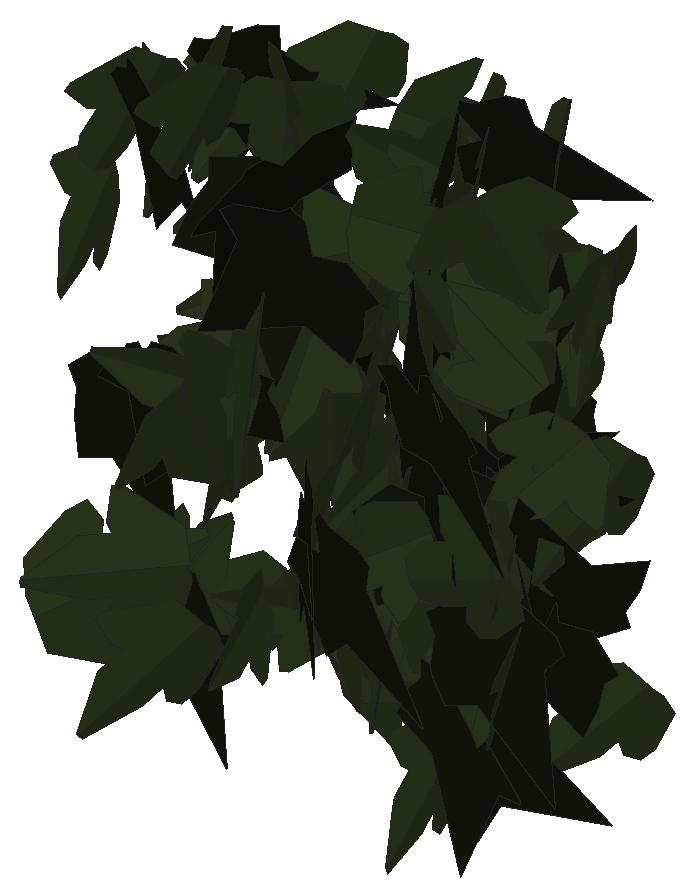
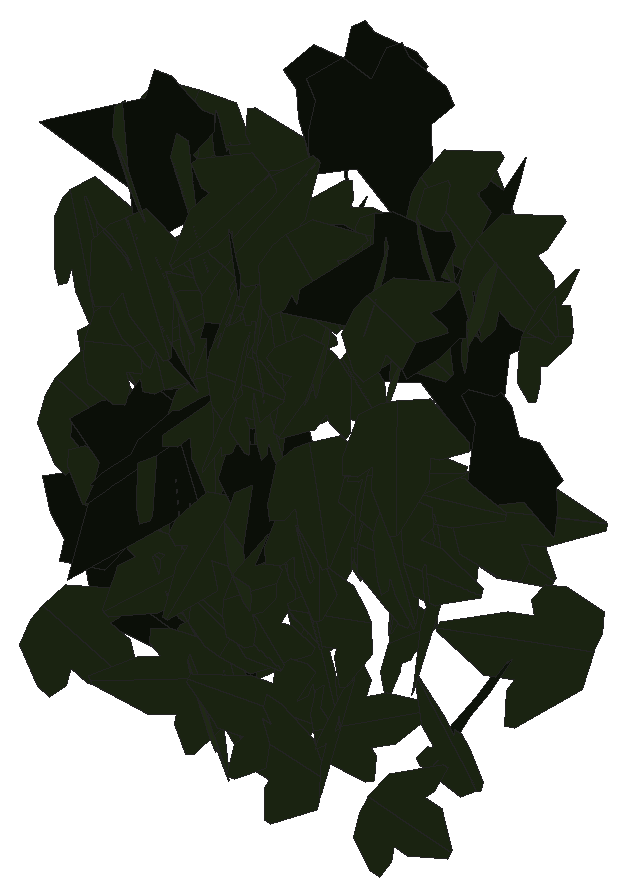
# SketchUp Ruby script. Lengths in inches.
U = 1.inch
M = Sketchup.active_model
def pt(a) = Geom::Point3d.new(a.map { |v| v * U })
def face(e, loops, mat)
  f = e.add_face(loops[0].map { |a| pt(a) })
  loops[1..].each { |l| e.add_face(l.map { |a| pt(a) }).erase! }
  f.material = f.back_material = mat if mat
  f
end
# faces: each face lists its corners as indices into pts; further lists are holes
def faces(e, pts, list, mat = nil) = list.each { |f| face(e, (f[0].is_a?(Array) ? f : [f]).map { |l| l.map { |i| pts[i] } }, mat) }
# xy, xz, yz: faces in a plane at the given z, y or x. An outline is a flat list of corners, or four numbers for a rectangle; further outlines are holes
def ring(l) = l.size == 4 ? [[l[0], l[1]], [l[2], l[1]], [l[2], l[3]], [l[0], l[3]]] : l.each_slice(2).to_a
def flat(e, list, mat, &to3) = list.each { |f| face(e, (f[0].is_a?(Array) ? f : [f]).map { |l| ring(l).map { |u, v| to3.(u, v) } }, mat) }
def xy(e, z, list, mat = nil) = flat(e, list, mat) { |x, y| [x, y, z] }
def xz(e, y, list, mat = nil) = flat(e, list, mat) { |x, z| [x, y, z] }
def yz(e, x, list, mat = nil) = flat(e, list, mat) { |y, z| [x, y, z] }
def lines(e, pts, list) = list.each { |a, b| e.add_line(pt(pts[a]), pt(pts[b])) }
# prism: a flat outline (further loops are holes) pulled along v
def prism(e, loops, v, mat = nil)
  f = face(e, loops, mat); d = Geom::Vector3d.new(v.map { |x| x * U })
  f.pushpull(f.normal.samedirection?(d) ? d.length : -d.length)
end
def box(e, o, s, mat = nil) = prism(e, [[o, [o[0] + s[0], o[1], o[2]], [o[0] + s[0], o[1] + s[1], o[2]], [o[0], o[1] + s[1], o[2]]]], [0, 0, s[2]], mat)
def at(x, y, z, deg = 0) = Geom::Transformation.translation(pt([x, y, z])) * Geom::Transformation.rotation(ORIGIN, Z_AXIS, deg.degrees)
def axes(o, x, y, z) = Geom::Transformation.new([*x, 0, *y, 0, *z, 0, *pt(o).to_a, 1])
def part(name) = M.definitions.add(name)
# library, detail: a bought-in or finely detailed component or shape, given as its bounding box
def library(name, o, s) = part(name).tap { |d| box(d.entities, o, s) }
def detail(e, o, s) = box(e.add_group.entities, o, s)
def put(e, d, t, mat = nil) = e.add_instance(d, t).tap { |i| i.material = mat if mat }
def group(e, t, mat = nil) = e.add_group.tap { |g| g.transformation = t; g.material = mat if mat }.entities
root = M.entities
M.materials.add("efeu1").color = [18, 25, 13]
M.materials.add("efeu2").color = [43, 57, 29]
c1 = part("ivyleaf_10")
p = [[0,0.5,-0.03],[-0.0625,2.02,-0.43],[-0.19,2.01,-0.46],[-0.54,1.05,-0.29],[-0.52,0.625,-0.18],[-0.83,0.76,-0.28],
  [-1.16,0.64,-0.33],[-1.15,0.33,-0.24],[-0.77,-0.39,0.02],[-0.3,-0.51,0.16],[0.04,-0.48,0.23],[-0.02,2.01,-0.4375],
  [-0.06,2.01,-0.43],[0.04,-0.49,0.23],[0.67,-0.49,0.14],[1.38,0.36,-0.2],[1.375,0.51,-0.24],[0.81,0.65,-0.19],
  [0.62,0.59,-0.15],[0.6,1.09,-0.28],[0.5,1.23,-0.31]]
faces(c1.entities,p,[[0,1,2,3,4,5,6,7,8,9,10],[11,12,0,13,14,15,16,17,18,19,20]],"efeu2")
c2 = part("ivyleaf_9")
p = [[1.54,2.16,1.25],[1.36,2.04,1.19],[-0.21,0.99,0.68],[-0.71,1.11,0.82],[-0.85,0.86,0.67],[-0.8,0.17,0.21],
  [-0.9,-0.01,0.1],[-0.67,-0.16,-0.02],[-0.08,-0.08,-0.05],[-0.03,-0.6,-0.4],[0.65,-0.88,-0.66],[0.83,-0.6,-0.49],
  [1.29,-0.42,-0.43],[1.8125,-0.07,-0.26],[1.21,0.44,0.15]]
faces(c2.entities,p,[[0,1,2,3,4,5,6,7,8,9,10,11,12,13,14]],"efeu1")
put(root,c1,axes([513.32,135.32,171.68],[-0.08732,-0.65374,0.43706],[-0.02249,-0.43749,-0.65888],[0.78606,-0.08514,0.0297]))
put(root,c1,axes([513.06,134.78,170.35],[-0.06101,-0.33846,0.66501],[0.36152,-0.5971,-0.27073],[0.65277,0.29906,0.21209]))
put(root,c1,axes([513.72,136.18,166.54],[-0.09693,0.07568,0.7615],[-0.51086,0.5651,-0.12118],[-0.56976,-0.51956,-0.02089]))
put(root,c1,axes([513.16,136.26,164.39],[0.50718,-0.21012,-0.38853],[0.35496,-0.15822,0.54892],[-0.2629,-0.619,-0.00842]))
put(root,c1,axes([513.18,136.01,170.99],[-0.24057,-0.00862,0.63768],[0.5315,-0.37936,0.19539],[0.35244,0.56621,0.14061]))
put(root,c1,axes([513.66,137.22,164],[-0.17056,-0.41151,0.50788],[-0.01949,-0.52144,-0.42905],[0.65338,-0.12298,0.11978]))
put(root,c1,axes([514.2,136.55,167.49],[0.09159,0.0185,-0.7632],[-0.75052,0.14293,-0.0866],[0.13978,0.75527,0.03508]))
put(root,c1,axes([513.24,133.97,165.2],[0.19421,0.17082,-0.85137],[0.64383,0.55707,0.25864],[0.58266,-0.67248,-0.00201]))
put(root,c1,axes([513.79,136.84,169.625],[-0.37954,-0.60035,-0.04],[0.01676,0.03673,-0.71024],[0.60145,-0.37987,-0.00545]))
put(root,c1,axes([514.01,136.83,171.28],[-0.35701,-0.40739,0.47497],[-0.10446,-0.50037,-0.50768],[0.61697,-0.32045,0.18889]))
put(root,c1,axes([513.93,136.76,167.95],[0.13667,-0.66248,0.06443],[0.01464,-0.06276,-0.67643],[0.66544,0.13745,0.00165]))
put(root,c1,axes([514.35,136.03,168.1],[-0.11845,-0.06289,0.67388],[-0.43804,-0.51439,-0.125],[0.51593,-0.45116,0.04858]))
put(root,c2,axes([513.64,135.52,164.69],[0.32318,-0.69175,0.08443],[0.0373,-0.07576,-0.76352],[0.69588,0.32532,0.00172]))
put(root,c1,axes([514.35,136.75,168.73],[0.0879,0.09809,-0.65288],[-0.4716,-0.4516,-0.13134],[-0.46203,0.47962,0.00986]))
put(root,c1,axes([514.0625,135.82,172.1],[0.3082,-0.50599,0.35522],[0.20219,-0.29258,-0.5922],[0.58423,0.36819,0.01756]))
put(root,c2,axes([513.78,136.0625,171.59],[0.13494,0.26931,-0.70933],[0.27273,0.65509,0.3006],[0.70802,-0.30367,0.0194]))
put(root,c2,axes([513.86,134.19,168.27],[-0.28502,-0.09388,-0.70569],[0.66464,0.23729,-0.30001],[0.2551,-0.72314,-0.00683]))
put(root,c2,axes([513.89,134.9,171.41],[0.08524,-0.47252,0.60804],[0.14853,-0.59018,-0.47946],[0.75559,0.16932,0.02566]))
put(root,c1,axes([514.42,136.36,169.05],[-0.25689,0.64643,0.18666],[-0.08928,0.16529,-0.69528],[-0.66689,-0.27114,0.02118]))
put(root,c1,axes([514.54,135.01,172.07],[-0.00408,-0.68886,0.41079],[0.01597,-0.41078,-0.68869],[0.80189,0.00468,0.0158]))
put(root,c1,axes([514.97,133.48,166.45],[-0.04546,-0.04195,0.78348],[-0.47666,-0.6219,-0.06095],[0.62322,-0.4787,0.01053]))
put(root,c1,axes([514.625,135.36,167.27],[0.1349,-0.53892,-0.51614],[-0.0178,0.52204,-0.54972],[0.746,0.10991,0.08022]))
put(root,c1,axes([514.82,136.28,171.54],[-0.52337,-0.46039,0.09507],[-0.06521,-0.06981,-0.69698],[0.46556,-0.52733,0.00926]))
put(root,c1,axes([515.08,136.48,164.51],[-0.13673,0.03474,-0.62065],[-0.56309,-0.27614,0.1086],[-0.26334,0.57241,0.09006]))
put(root,c1,axes([514.47,135.98,170.16],[-0.25384,0.46249,-0.49972],[0.2253,-0.44622,-0.52742],[-0.64254,-0.33918,0.01248]))
put(root,c1,axes([514.51,136.41,171.78],[-0.41464,0.50002,-0.3271],[0.21653,-0.24533,-0.64952],[-0.55689,-0.46769,-0.009]))
put(root,c1,axes([514.95,136.55,164.92],[-0.29166,0.60031,0.10335],[-0.0587,0.08635,-0.66724],[-0.6063,-0.29713,0.01489]))
put(root,c1,axes([514.53,136.92,166.48],[-0.20723,0.09072,-0.63142],[0.56466,-0.2828,-0.22595],[-0.29679,-0.60139,0.011]))
put(root,c1,axes([515.11,136.86,167.78],[-0.40097,-0.54568,-0.01251],[0.00994,0.00822,-0.67715],[0.54573,-0.40108,0.00314]))
put(root,c1,axes([515.16,136.9,168.5625],[-0.30215,-0.6049,0.05545],[-0.02207,-0.05096,-0.67616],[0.60704,-0.30294,0.00301]))
put(root,c1,axes([515.2,137.2,171.93],[-0.29718,-0.49884,0.3104],[-0.05496,-0.32272,-0.57126],[0.58495,-0.28376,0.10402]))
put(root,c1,axes([515.21,135.11,165.18],[-0.03071,0.2233,-0.60377],[-0.00677,-0.60453,-0.22324],[-0.6437,-0.0043,0.03115]))
put(root,c1,axes([515.7,136.23,165.4375],[-0.32304,0.10404,0.5461],[-0.51564,0.17997,-0.33931],[-0.20776,-0.60844,-0.00699]))
put(root,c2,axes([515.59,133.45,169.28],[0.32299,0.46235,-0.55271],[-0.34821,-0.43013,-0.5633],[-0.63087,0.47412,0.02794]))
put(root,c1,axes([515.45,136.24,167.52],[-0.11325,-0.62591,-0.07851],[0.0108,0.07783,-0.63607],[0.63073,-0.11372,-0.0032]))
put(root,c1,axes([515.71,132.97,165.87],[-0.18062,-0.49797,0.59155],[-0.21017,-0.55299,-0.52968],[0.74413,-0.27705,-0.00602]))
put(root,c1,axes([515.31,136.57,169.84],[-0.57023,0.08825,-0.28166],[0.27161,-0.08298,-0.57587],[-0.11555,-0.63057,0.03637]))
put(root,c1,axes([515.65,136.75,167.36],[0.46985,-0.55043,-0.28111],[-0.18585,0.21094,-0.72368],[0.58945,0.50525,-0.00411]))
put(root,c1,axes([515.5625,136.34,170.16],[-0.47216,0.42684,-0.06049],[0.04122,-0.0446,-0.63647],[-0.42913,-0.47392,0.00542]))
put(root,c1,axes([516.16,133.28,169.33],[-0.20729,0.04473,-0.76954],[-0.74755,-0.20609,0.18938],[-0.18807,0.76986,0.09541]))
put(root,c2,axes([515.62,135.06,171.03],[-0.44138,-0.52209,-0.37281],[0.2329,0.29124,-0.6836],[0.59776,-0.49898,-0.00893]))
put(root,c1,axes([515.98,135.15,169.04],[0.21101,0.533,-0.30857],[-0.14739,-0.273,-0.57234],[-0.59798,0.25537,0.03218]))
put(root,c1,axes([515.54,136.78,163.85],[0.07508,-0.00656,-0.7683],[0.72273,-0.26137,0.07286],[-0.26074,-0.72636,-0.01928]))
put(root,c1,axes([515.95,136.4,166.77],[0.5732,-0.198,0.21383],[0.20355,-0.06563,-0.60641],[0.20855,0.60825,0.00417]))
put(root,c1,axes([516.05,137.36,166.48],[-0.03952,-0.15495,0.62079],[0.22707,-0.58488,-0.13153],[0.59818,0.21178,0.09095]))
put(root,c1,axes([516.17,135.27,167.16],[0.32619,-0.64833,0.21678],[0.1042,-0.19024,-0.72573],[0.67563,0.34236,0.00727]))
put(root,c1,axes([516.24,136.51,169.08],[0.16798,-0.62768,0.07538],[0.0277,-0.07061,-0.64971],[0.63158,0.17004,0.00844]))
put(root,c1,axes([516.5,135.98,169.89],[-0.58682,-0.11813,0.23916],[-0.2272,-0.08145,-0.59771],[0.13976,-0.62843,0.03251]))
put(root,c2,axes([515.68,136.8,167.73],[0.3406,-0.33455,0.60485],[0.41726,-0.43806,-0.47726],[0.55105,0.53848,-0.01247]))
put(root,c1,axes([515.9,136.45,164.3],[0.28401,0.23927,-0.69912],[0.54287,0.44057,0.37132],[0.50131,-0.61264,-0.00601]))
put(root,c1,axes([516.31,136.36,167.06],[0.04832,0.1535,-0.66955],[-0.12338,-0.65835,-0.15984],[-0.67575,0.13118,-0.01869]))
put(root,c1,axes([516.62,136.77,165.52],[-0.60869,-0.21908,-0.35197],[-0.31753,-0.15565,0.64601],[-0.26655,0.68568,0.03419]))
put(root,c1,axes([516.89,136.59,169.25],[-0.10985,0.12575,-0.71735],[-0.59963,0.39611,0.16126],[0.41333,0.60807,0.0433]))
put(root,c1,axes([516.3,137.07,167.19],[0.26297,-0.52173,0.42454],[0.19984,-0.37465,-0.5842],[0.64227,0.33019,0.00795]))
put(root,c1,axes([516.0625,136.95,170.03],[0.1598,-0.21747,0.57718],[0.49507,-0.31039,-0.25402],[0.36787,0.51218,0.09113]))
put(root,c1,axes([516.73,134.9,170.74],[-0.10812,0.0104,0.6499],[-0.25929,-0.60483,-0.03346],[0.59603,-0.26123,0.10333]))
put(root,c2,axes([516.75,133.65,172.41],[-0.16706,0.76038,-0.38991],[0.0861,-0.38029,-0.77851],[-0.85017,-0.18793,-0.00223]))
put(root,c1,axes([516.11,135.8125,164.99],[0.05625,-0.17617,-0.67575],[0.4576,-0.50281,0.16917],[-0.52751,-0.45496,0.0747]))
put(root,c1,axes([516.625,135.84,170.07],[-0.0733,-0.4451,-0.52544],[0.06645,0.52137,-0.45092],[0.68541,-0.09814,-0.01248]))
put(root,c1,axes([516.85,136.34,171.18],[-0.34196,-0.32832,-0.55329],[-0.36296,-0.4189,0.4729],[-0.53121,0.49758,0.03305]))
put(root,c1,axes([517.04,136.85,165.92],[0.3153,-0.08677,-0.62442],[-0.60282,0.16283,-0.32702],[0.1845,0.68029,-0.00137]))
put(root,c1,axes([516.46,136.08,165.27],[0.45508,-0.45276,0.36218],[0.27211,-0.23978,-0.64166],[0.51198,0.52989,0.0191]))
put(root,c1,axes([516.71,131.88,170.02],[-0.13923,-0.78876,-0.40578],[0.08955,0.39615,-0.80077],[0.88249,-0.16464,0.01724]))
put(root,c1,axes([516.8,136.57,168.82],[-0.12962,0.55616,-0.33098],[0.07246,-0.32296,-0.57106],[-0.64312,-0.14848,0.00237]))
put(root,c1,axes([516.84,135.18,166.67],[0.04433,0.74047,-0.08975],[-0.01158,-0.08921,-0.74177],[-0.7458,0.0454,0.00618]))
put(root,c1,axes([516.8,136.28,171.96],[0.11677,0.32998,0.59583],[0.04612,0.5993,-0.34094],[-0.67954,0.09737,0.07924]))
put(root,c1,axes([516.92,136.64,166.96],[-0.23638,-0.46721,-0.47243],[0.20385,0.42625,-0.52354],[0.63239,-0.31204,-0.00782]))
put(root,c1,axes([517.32,135.63,166.64],[-0.48158,0.17381,0.41087],[-0.41249,0.05681,-0.50751],[-0.16993,-0.63048,0.06754]))
put(root,c1,axes([516.89,135.52,166.38],[0.1384,-0.66648,-0.11301],[0.06007,-0.10277,0.67967],[-0.67332,-0.14616,0.03741]))
put(root,c1,axes([517.05,136.78,170.75],[-0.06739,-0.12145,-0.66567],[-0.02525,-0.66804,0.12444],[-0.67618,0.03705,0.06169]))
put(root,c1,axes([517.11,136.875,164.58],[0.41376,-0.60576,0.09546],[0.04031,-0.08804,-0.7334],[0.61191,0.4154,-0.01623]))
put(root,c1,axes([516.98,136.31,164.37],[0.34166,-0.49758,0.39293],[0.27384,-0.28676,-0.60125],[0.57183,0.43462,0.05315]))
put(root,c1,axes([517.15,136.09,170.34],[-0.32354,0.56651,-0.06615],[0.02827,-0.06003,-0.65237],[-0.56966,-0.32473,0.00519]))
put(root,c1,axes([517.46,136.1875,168.47],[-0.35983,-0.54915,-0.00647],[0.00405,0.00508,-0.65654],[0.54918,-0.35985,0.0006]))
put(root,c2,axes([517.87,132.78,171.97],[0.14546,0.2147,-0.77453],[-0.61022,-0.48277,-0.24843],[-0.52309,0.62289,0.07443]))
put(root,c1,axes([517.51,134.47,169.38],[0.26921,-0.70867,-0.2343],[-0.06834,0.22463,-0.75793],[0.74326,0.27734,0.01517]))
put(root,c2,axes([517.86,135.37,171.67],[-0.15495,0.04401,-0.79776],[-0.74645,0.28179,0.16053],[0.2849,0.76225,-0.01329]))
put(root,c1,axes([517.17,132.56,170.8],[0.59668,-0.55738,0.47425],[0.38498,-0.28134,-0.81501],[0.62239,0.70837,0.04947]))
put(root,c1,axes([517.09,136.125,165.26],[0.45091,0.17818,-0.53629],[0.48671,0.22619,0.48438],[0.28717,-0.66315,0.02112]))
put(root,c1,axes([517.9,136.41,169.78],[0.20776,0.02341,0.63738],[-0.56306,0.32162,0.17172],[-0.2996,-0.5882,0.11926]))
put(root,c1,axes([517.5,136.76,172.12],[0.44241,-0.57961,0.13419],[0.09192,-0.09863,-0.72905],[0.5878,0.45167,0.01301]))
put(root,c2,axes([517.4,135.92,170.33],[0.00177,0.03083,-0.81568],[0.64375,-0.50157,-0.01757],[-0.50187,-0.64325,-0.0254]))
put(root,c1,axes([517.15,136.77,164.58],[-0.13005,-0.0602,-0.75149],[0.73921,0.13965,-0.13911],[0.14813,-0.74977,0.03443]))
put(root,c1,axes([517.43,136.75,166.26],[-0.26445,0.16571,0.61709],[0.52927,-0.31735,0.31203],[0.35797,0.59163,-0.00547]))
put(root,c1,axes([517.61,135.52,165.96],[-0.13296,-0.31212,-0.56424],[0.32613,0.46444,-0.33377],[0.55626,-0.3469,0.06081]))
put(root,c1,axes([518.08,134.375,167.44],[0.11546,0.10985,-0.6521],[-0.45889,-0.46333,-0.1593],[-0.47616,0.47317,-0.0046]))
put(root,c1,axes([517.4,134.71,171.43],[0.0773,0.08817,0.65436],[0.47498,0.45022,-0.11677],[-0.45865,0.48111,-0.01065]))
put(root,c2,axes([517.39,135.42,168.54],[-0.08414,-0.06326,-0.801],[0.80308,-0.03262,-0.08178],[-0.02594,-0.80475,0.06628]))
put(root,c1,axes([517.29,135.92,169.8],[0.04842,-0.13103,-0.80215],[0.81272,0.01812,0.0461],[0.01043,-0.80341,0.13187]))
put(root,c2,axes([517.85,137.38,168.07],[-0.16877,-0.72254,0.32211],[-0.02878,-0.32353,-0.74081],[0.79056,-0.16602,0.04179]))
put(root,c1,axes([518.39,136.25,169.11],[0.41054,0.32726,0.60215],[-0.50171,-0.33465,0.52395],[0.46687,-0.64741,0.03355]))
put(root,c1,axes([518.43,136.73,170.73],[-0.61078,-0.01599,0.45563],[-0.45506,-0.02519,-0.61089],[0.02788,-0.76159,0.01064]))
put(root,c1,axes([518.12,136.39,167.4],[-0.00198,-0.71401,0.02879],[-0.00028,-0.02879,-0.71401],[0.71459,-0.00199,-0.0002]))
put(root,c1,axes([517.98,135.2,164.1],[-0.0261,-0.41174,0.64745],[0.25272,-0.61629,-0.38174],[0.72447,0.20015,0.15649]))
put(root,c1,axes([517.64,136.7,166.03],[0.42135,0.17662,0.56812],[0.52508,0.21693,-0.45687],[-0.27973,0.67323,-0.00183]))
put(root,c2,axes([518.12,136.24,167.57],[0.44095,0.61111,0.25887],[0.14899,0.21171,-0.75358],[-0.64674,0.46543,0.0029]))
put(root,c1,axes([517.86,135.01,170.67],[-0.06942,-0.02924,-0.7553],[0.48663,-0.58211,-0.02219],[-0.57838,-0.48626,0.07199]))
put(root,c2,axes([517.67,136.27,166.96],[0.2267,-0.16259,0.72341],[0.71897,-0.13668,-0.25602],[0.18121,0.74567,0.11081]))
put(root,c2,axes([517.89,135.15,167.54],[-0.16678,-0.29222,-0.73956],[0.45108,0.58754,-0.33388],[0.65487,-0.47912,0.04163]))
put(root,c2,axes([518.9375,136.125,169.68],[-0.33871,0.01213,-0.73003],[-0.72915,0.03596,0.3389],[0.03772,0.80397,-0.00415]))
put(root,c2,axes([518.98,136.08,165.89],[0.1226,0.11441,-0.79143],[-0.63668,-0.47048,-0.16664],[-0.48383,0.6481,0.01875]))
put(root,c2,axes([517.92,136.17,172.09],[0.34323,0.18713,-0.67012],[0.54545,0.3915,0.38871],[0.43193,-0.64311,0.04164]))
put(root,c1,axes([518.78,135.72,169.53],[0.22256,0.55719,0.38691],[-0.20463,-0.33308,0.59738],[0.64674,-0.29713,0.05587]))
put(root,c1,axes([518.36,136.16,168.77],[-0.62635,-0.02502,0.39526],[0.39604,-0.04365,0.62483],[0.00218,0.73935,0.05026]))
put(root,c2,axes([518.17,134.57,169.33],[0.50452,-0.6398,0.07736],[0.0428,-0.06476,-0.81476],[0.64304,0.50629,-0.00646]))
put(root,c1,axes([518.61,135.27,165.74],[0.66597,0.04095,-0.03859],[-0.03851,-0.00251,-0.66722],[-0.04103,0.66708,-0.00014]))
put(root,c1,axes([518.5,136.79,172.2],[0.46035,-0.45205,0.31976],[0.24406,-0.2076,-0.64487],[0.49702,0.52064,0.02049]))
put(root,c1,axes([519.27,134.47,167.35],[-0.22481,-0.07761,0.73543],[-0.70497,-0.20971,-0.23762],[0.2234,-0.73988,-0.00979]))
put(root,c2,axes([518.3,132.17,168.9],[-0.0211,-0.1428,-0.81049],[0.79897,-0.19793,0.01407],[-0.19731,-0.78623,0.14366]))
put(root,c2,axes([518.46,135.07,164.82],[0.07631,-0.69201,0.33747],[0.07374,-0.33099,-0.69541],[0.76637,0.10075,0.03331]))
put(root,c1,axes([518.76,135.12,171.84],[-0.55658,-0.53977,-0.29898],[0.21884,0.20379,-0.77531],[0.57693,-0.59803,0.00565]))
put(root,c2,axes([518.18,135.22,164.5],[0.2377,-0.03307,-0.74369],[0.59458,0.47819,0.16877],[0.44793,-0.61718,0.17062]))
put(root,c1,axes([518.8125,136.5,166.87],[-0.23979,-0.59809,-0.16156],[-0.05925,-0.1503,0.64437],[-0.61669,0.247,0.00091]))
put(root,c1,axes([518.86,136.7,169.07],[0.0293,-0.2607,0.61197],[0.03241,-0.61128,-0.26196],[0.6644,0.04131,-0.01421]))
put(root,c1,axes([518.85,135.79,167.35],[-0.03695,0.6081,0.31425],[-0.05822,0.31078,-0.60823],[-0.68202,-0.05947,0.03489]))
put(root,c2,axes([518.9,136.11,165.9],[0.56366,0.27199,0.51151],[-0.47864,-0.18343,0.62498],[0.32638,-0.73872,0.03315]))
put(root,c2,axes([518.68,132.0625,168.43],[0.58341,-0.50657,-0.29355],[-0.20109,0.21582,-0.7721],[0.54986,0.61641,0.02909]))
put(root,c1,axes([519.07,135.28,166.06],[0.34468,-0.5933,0.12863],[0.05361,-0.1176,-0.68605],[0.60472,0.3486,-0.0125]))
put(root,c1,axes([519.45,136.9,164.65],[-0.31344,-0.36843,0.52897],[-0.31052,-0.42916,-0.48291],[0.56492,-0.44032,0.02806]))
put(root,c1,axes([519.46,135.68,168.59],[0.49255,0.14793,-0.44104],[-0.43355,-0.08688,-0.51332],[-0.16864,0.65543,0.03151]))
put(root,c2,axes([518.88,134.96,166.3],[-0.31504,-0.15948,-0.69624],[0.60205,0.35017,-0.35263],[0.38434,-0.67925,-0.01832]))
put(root,c1,axes([518.97,135.21,167.31],[-0.01526,-0.09309,0.66356],[0.44761,-0.49533,-0.0592],[0.49862,0.44181,0.07345]))
put(root,c1,axes([519.07,136.48,170.51],[0.65476,-0.27926,0.25449],[0.23882,-0.08867,-0.71173],[0.29278,0.69686,0.01142]))
put(root,c1,axes([519.43,136.56,170.73],[0.07717,-0.77849,-0.02033],[-0.0014,0.02029,-0.7823],[0.77875,0.07718,0.00061]))
put(root,c1,axes([519.54,136.49,167.95],[-0.15316,-0.5542,0.51689],[-0.06026,-0.51676,-0.57192],[0.75543,-0.15358,0.05917]))
